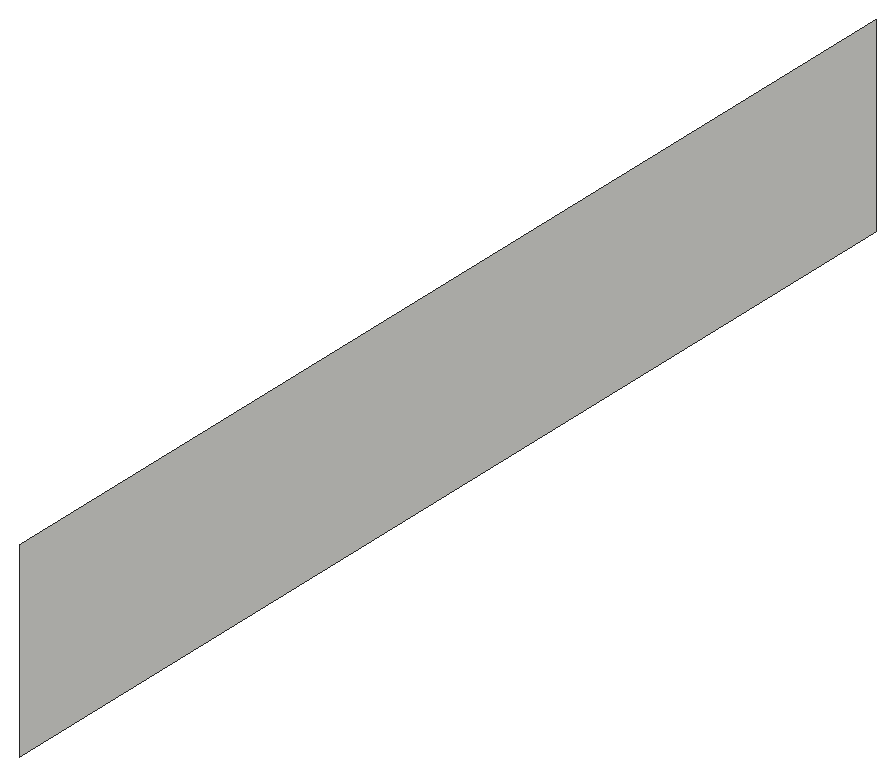
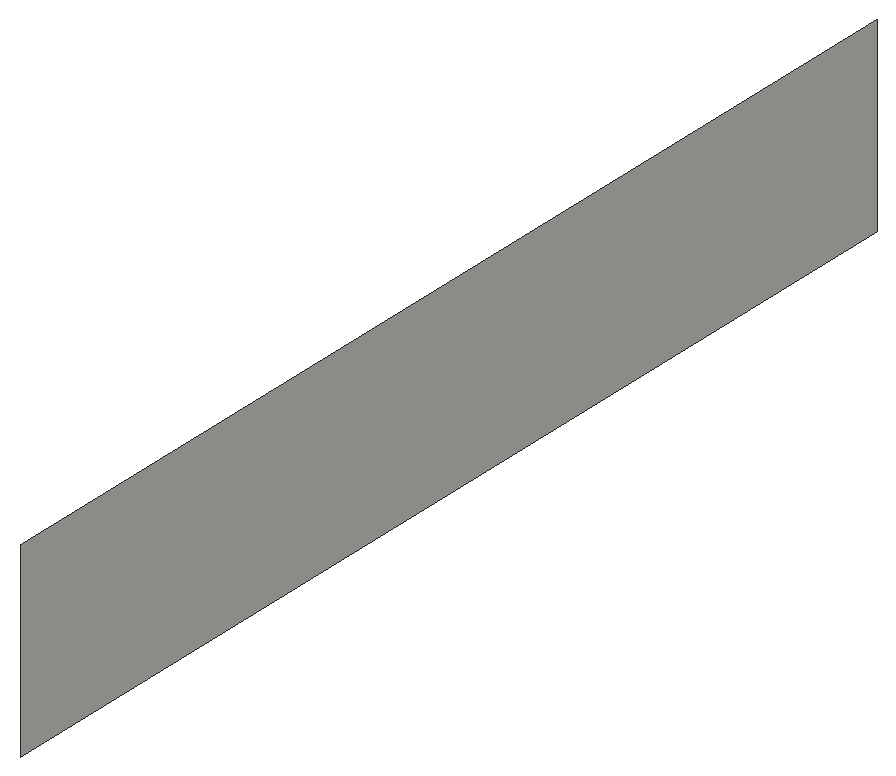
# SketchUp Ruby script. Lengths in inches.
U = 1.inch
M = Sketchup.active_model
def pt(a) = Geom::Point3d.new(a.map { |v| v * U })
def face(e, loops, mat)
  f = e.add_face(loops[0].map { |a| pt(a) })
  loops[1..].each { |l| e.add_face(l.map { |a| pt(a) }).erase! }
  f.material = f.back_material = mat if mat
  f
end
# faces: each face lists its corners as indices into pts; further lists are holes
def faces(e, pts, list, mat = nil) = list.each { |f| face(e, (f[0].is_a?(Array) ? f : [f]).map { |l| l.map { |i| pts[i] } }, mat) }
# xy, xz, yz: faces in a plane at the given z, y or x. An outline is a flat list of corners, or four numbers for a rectangle; further outlines are holes
def ring(l) = l.size == 4 ? [[l[0], l[1]], [l[2], l[1]], [l[2], l[3]], [l[0], l[3]]] : l.each_slice(2).to_a
def flat(e, list, mat, &to3) = list.each { |f| face(e, (f[0].is_a?(Array) ? f : [f]).map { |l| ring(l).map { |u, v| to3.(u, v) } }, mat) }
def xy(e, z, list, mat = nil) = flat(e, list, mat) { |x, y| [x, y, z] }
def xz(e, y, list, mat = nil) = flat(e, list, mat) { |x, z| [x, y, z] }
def yz(e, x, list, mat = nil) = flat(e, list, mat) { |y, z| [x, y, z] }
def lines(e, pts, list) = list.each { |a, b| e.add_line(pt(pts[a]), pt(pts[b])) }
# prism: a flat outline (further loops are holes) pulled along v
def prism(e, loops, v, mat = nil)
  f = face(e, loops, mat); d = Geom::Vector3d.new(v.map { |x| x * U })
  f.pushpull(f.normal.samedirection?(d) ? d.length : -d.length)
end
def box(e, o, s, mat = nil) = prism(e, [[o, [o[0] + s[0], o[1], o[2]], [o[0] + s[0], o[1] + s[1], o[2]], [o[0], o[1] + s[1], o[2]]]], [0, 0, s[2]], mat)
def at(x, y, z, deg = 0) = Geom::Transformation.translation(pt([x, y, z])) * Geom::Transformation.rotation(ORIGIN, Z_AXIS, deg.degrees)
def axes(o, x, y, z) = Geom::Transformation.new([*x, 0, *y, 0, *z, 0, *pt(o).to_a, 1])
def part(name) = M.definitions.add(name)
# library, detail: a bought-in or finely detailed component or shape, given as its bounding box
def library(name, o, s) = part(name).tap { |d| box(d.entities, o, s) }
def detail(e, o, s) = box(e.add_group.entities, o, s)
def put(e, d, t, mat = nil) = e.add_instance(d, t).tap { |i| i.material = mat if mat }
def group(e, t, mat = nil) = e.add_group.tap { |g| g.transformation = t; g.material = mat if mat }.entities
root = M.entities
yz(root,189.49,[[199.23,95.36,219.06,98.875]])
